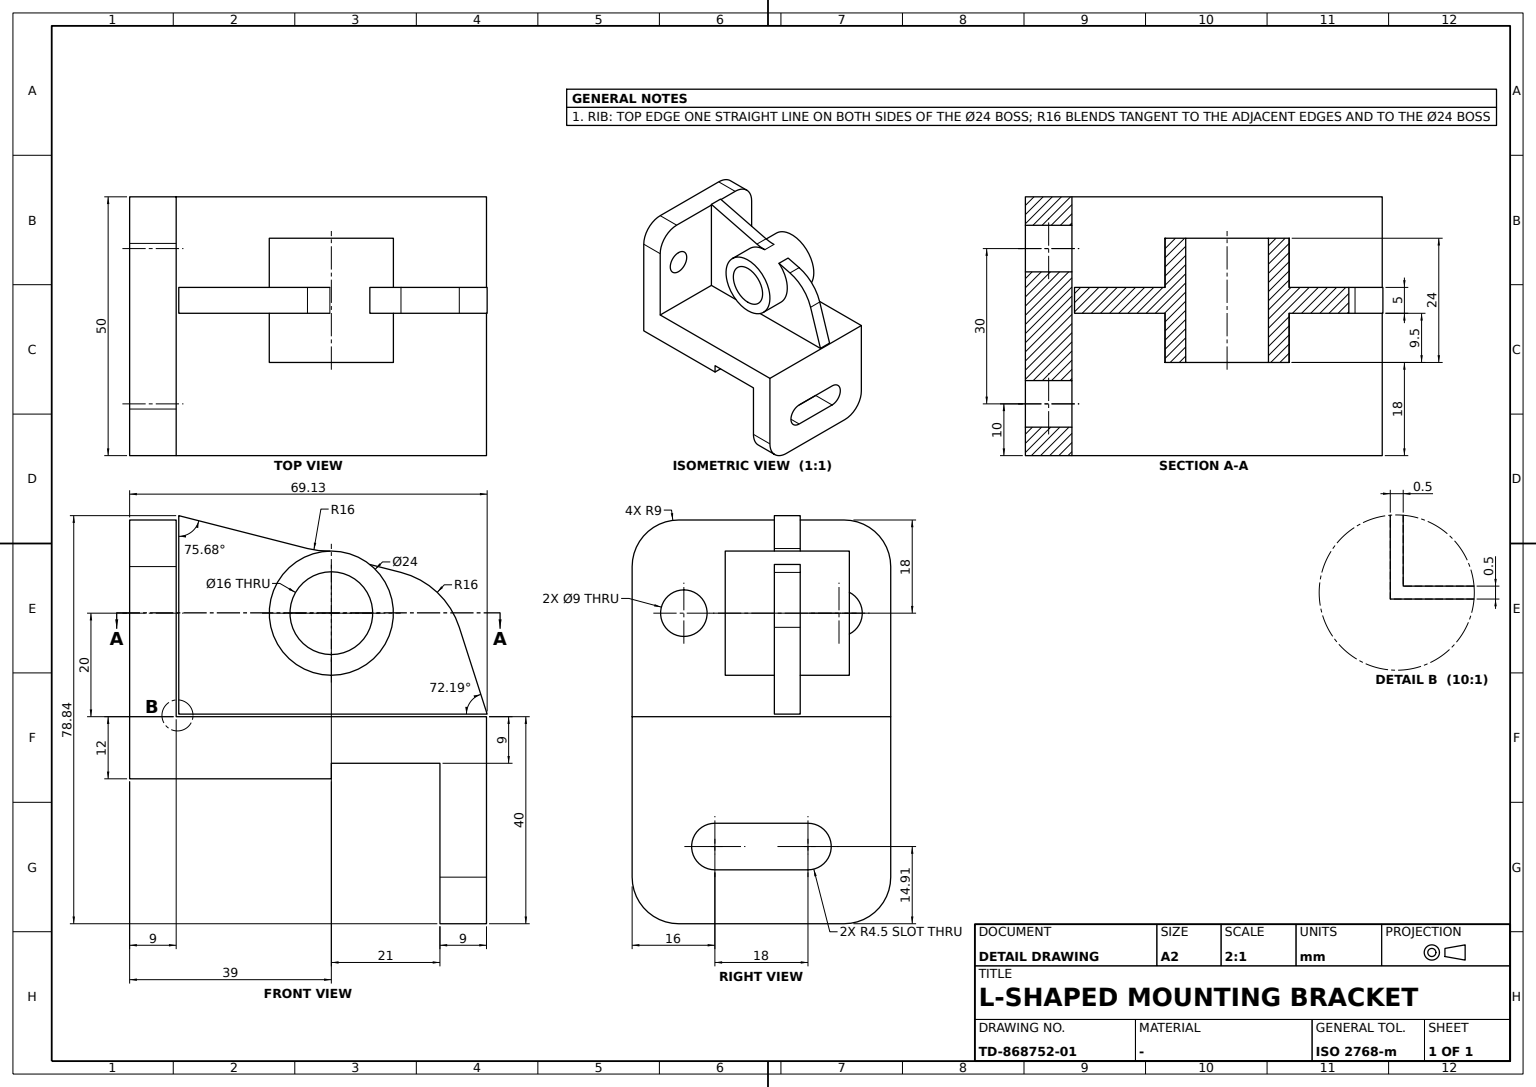
ISO-10303-21;
HEADER;
FILE_DESCRIPTION((''),'2;1');
FILE_NAME('','',(''),(''),'','','');
FILE_SCHEMA(('AUTOMOTIVE_DESIGN'));
ENDSEC;
DATA;
#1=APPLICATION_CONTEXT('');
#2=PRODUCT_CONTEXT('',#1,'mechanical');
#3=PRODUCT('','','',(#2));
#4=PRODUCT_DEFINITION_FORMATION('','',#3);
#5=PRODUCT_DEFINITION_CONTEXT('',#1,'design');
#6=PRODUCT_DEFINITION('','',#4,#5);
#7=PRODUCT_DEFINITION_SHAPE('','',#6);
#8=(LENGTH_UNIT()NAMED_UNIT(*)SI_UNIT(.MILLI.,.METRE.));
#9=(NAMED_UNIT(*)PLANE_ANGLE_UNIT()SI_UNIT($,.RADIAN.));
#10=(NAMED_UNIT(*)SI_UNIT($,.STERADIAN.)SOLID_ANGLE_UNIT());
#11=UNCERTAINTY_MEASURE_WITH_UNIT(LENGTH_MEASURE(0.005),#8,'distance_accuracy_value','');
#12=(GEOMETRIC_REPRESENTATION_CONTEXT(3)GLOBAL_UNCERTAINTY_ASSIGNED_CONTEXT((#11))GLOBAL_UNIT_ASSIGNED_CONTEXT((#8,#9,#10))REPRESENTATION_CONTEXT('',''));
#13=CARTESIAN_POINT('',(0.,-51.,12.));
#14=VERTEX_POINT('',#13);
#15=CARTESIAN_POINT('',(0.,-51.,41.));
#16=VERTEX_POINT('',#15);
#17=CARTESIAN_POINT('',(0.,-51.,0.));
#18=DIRECTION('',(0.,0.,1.));
#19=VECTOR('',#18,1000.);
#20=LINE('',#17,#19);
#21=EDGE_CURVE('',#14,#16,#20,.T.);
#22=ORIENTED_EDGE('',*,*,#21,.T.);
#23=CARTESIAN_POINT('',(9.,-51.,50.));
#24=VERTEX_POINT('',#23);
#25=CARTESIAN_POINT('',(9.,-51.,41.));
#26=DIRECTION('',(0.,1.,0.));
#27=AXIS2_PLACEMENT_3D('',#25,#26,#18);
#28=CIRCLE('',#27,9.);
#29=EDGE_CURVE('',#16,#24,#28,.T.);
#30=ORIENTED_EDGE('',*,*,#29,.T.);
#31=CARTESIAN_POINT('',(41.,-51.,50.));
#32=VERTEX_POINT('',#31);
#33=CARTESIAN_POINT('',(0.,-51.,50.));
#34=DIRECTION('',(1.,0.,0.));
#35=VECTOR('',#34,1000.);
#36=LINE('',#33,#35);
#37=EDGE_CURVE('',#24,#32,#36,.T.);
#38=ORIENTED_EDGE('',*,*,#37,.T.);
#39=CARTESIAN_POINT('',(50.,-51.,41.));
#40=VERTEX_POINT('',#39);
#41=CARTESIAN_POINT('',(41.,-51.,41.));
#42=AXIS2_PLACEMENT_3D('',#41,#26,#18);
#43=CIRCLE('',#42,9.);
#44=EDGE_CURVE('',#32,#40,#43,.T.);
#45=ORIENTED_EDGE('',*,*,#44,.T.);
#46=CARTESIAN_POINT('',(50.,-51.,12.));
#47=VERTEX_POINT('',#46);
#48=CARTESIAN_POINT('',(50.,-51.,0.));
#49=LINE('',#48,#19);
#50=EDGE_CURVE('',#47,#40,#49,.T.);
#51=ORIENTED_EDGE('',*,*,#50,.F.);
#52=LINE('',#13,#35);
#53=EDGE_CURVE('',#14,#47,#52,.T.);
#54=ORIENTED_EDGE('',*,*,#53,.F.);
#55=EDGE_LOOP('',(#22,#30,#38,#45,#51,#54));
#56=FACE_BOUND('',#55,.T.);
#57=CARTESIAN_POINT('',(10.,-51.,36.5));
#58=VERTEX_POINT('',#57);
#59=CARTESIAN_POINT('',(10.,-51.,32.));
#60=AXIS2_PLACEMENT_3D('',#59,#26,#18);
#61=CIRCLE('',#60,4.5);
#62=EDGE_CURVE('',#58,#58,#61,.T.);
#63=ORIENTED_EDGE('',*,*,#62,.F.);
#64=EDGE_LOOP('',(#63));
#65=FACE_BOUND('',#64,.T.);
#66=CARTESIAN_POINT('',(40.,-51.,36.5));
#67=VERTEX_POINT('',#66);
#68=CARTESIAN_POINT('',(40.,-51.,32.));
#69=AXIS2_PLACEMENT_3D('',#68,#26,#18);
#70=CIRCLE('',#69,4.5);
#71=EDGE_CURVE('',#67,#67,#70,.T.);
#72=ORIENTED_EDGE('',*,*,#71,.F.);
#73=EDGE_LOOP('',(#72));
#74=FACE_BOUND('',#73,.T.);
#75=AXIS2_PLACEMENT_3D('',#13,#26,#18);
#76=PLANE('',#75);
#77=ADVANCED_FACE('',(#56,#65,#74),#76,.T.);
#78=CARTESIAN_POINT('',(34.,9.,-8.585905426));
#79=VERTEX_POINT('',#78);
#80=CARTESIAN_POINT('',(34.,0.,-8.585905426));
#81=VERTEX_POINT('',#80);
#82=CARTESIAN_POINT('',(34.,-26.16,-8.585905426));
#83=VECTOR('',#26,1000.);
#84=LINE('',#82,#83);
#85=EDGE_CURVE('',#79,#81,#84,.F.);
#86=ORIENTED_EDGE('',*,*,#85,.F.);
#87=CARTESIAN_POINT('',(34.,9.,-17.585905426));
#88=VERTEX_POINT('',#87);
#89=CARTESIAN_POINT('',(34.,9.,-13.085905426));
#90=AXIS2_PLACEMENT_3D('',#89,#26,#18);
#91=CIRCLE('',#90,4.5);
#92=EDGE_CURVE('',#79,#88,#91,.T.);
#93=ORIENTED_EDGE('',*,*,#92,.T.);
#94=CARTESIAN_POINT('',(34.,0.,-17.585905426));
#95=VERTEX_POINT('',#94);
#96=CARTESIAN_POINT('',(34.,-26.16,-17.585905426));
#97=LINE('',#96,#83);
#98=EDGE_CURVE('',#88,#95,#97,.F.);
#99=ORIENTED_EDGE('',*,*,#98,.T.);
#100=CARTESIAN_POINT('',(34.,0.,-13.085905426));
#101=DIRECTION('',(0.,-1.,0.));
#102=DIRECTION('',(0.,0.,-1.));
#103=AXIS2_PLACEMENT_3D('',#100,#101,#102);
#104=CIRCLE('',#103,4.5);
#105=EDGE_CURVE('',#95,#81,#104,.T.);
#106=ORIENTED_EDGE('',*,*,#105,.T.);
#107=EDGE_LOOP('',(#86,#93,#99,#106));
#108=FACE_BOUND('',#107,.T.);
#109=CARTESIAN_POINT('',(34.,-26.16,-13.085905426));
#110=DIRECTION('',(-1.,0.,0.));
#111=AXIS2_PLACEMENT_3D('',#109,#26,#110);
#112=CYLINDRICAL_SURFACE('',#111,4.5);
#113=ADVANCED_FACE('',(#108),#112,.F.);
#114=ORIENTED_EDGE('',*,*,#62,.T.);
#115=EDGE_LOOP('',(#114));
#116=FACE_BOUND('',#115,.T.);
#117=CARTESIAN_POINT('',(10.,-60.,27.5));
#118=VERTEX_POINT('',#117);
#119=CARTESIAN_POINT('',(10.,-60.,32.));
#120=AXIS2_PLACEMENT_3D('',#119,#101,#102);
#121=CIRCLE('',#120,4.5);
#122=EDGE_CURVE('',#118,#118,#121,.T.);
#123=ORIENTED_EDGE('',*,*,#122,.T.);
#124=EDGE_LOOP('',(#123));
#125=FACE_BOUND('',#124,.T.);
#126=CARTESIAN_POINT('',(10.,-56.160000001,32.));
#127=AXIS2_PLACEMENT_3D('',#126,#26,#110);
#128=CYLINDRICAL_SURFACE('',#127,4.5);
#129=ADVANCED_FACE('',(#116,#125),#128,.F.);
#130=CARTESIAN_POINT('',(0.,-21.,3.));
#131=VERTEX_POINT('',#130);
#132=CARTESIAN_POINT('',(0.,0.,3.));
#133=VERTEX_POINT('',#132);
#134=LINE('',#132,#83);
#135=EDGE_CURVE('',#131,#133,#134,.T.);
#136=ORIENTED_EDGE('',*,*,#135,.T.);
#137=CARTESIAN_POINT('',(50.,0.,3.));
#138=VERTEX_POINT('',#137);
#139=LINE('',#132,#35);
#140=EDGE_CURVE('',#133,#138,#139,.T.);
#141=ORIENTED_EDGE('',*,*,#140,.T.);
#142=CARTESIAN_POINT('',(50.,-21.,3.));
#143=VERTEX_POINT('',#142);
#144=LINE('',#137,#83);
#145=EDGE_CURVE('',#143,#138,#144,.T.);
#146=ORIENTED_EDGE('',*,*,#145,.F.);
#147=LINE('',#130,#35);
#148=EDGE_CURVE('',#131,#143,#147,.T.);
#149=ORIENTED_EDGE('',*,*,#148,.F.);
#150=EDGE_LOOP('',(#136,#141,#146,#149));
#151=FACE_BOUND('',#150,.T.);
#152=AXIS2_PLACEMENT_3D('',#130,#102,#26);
#153=PLANE('',#152);
#154=ADVANCED_FACE('',(#151),#153,.T.);
#155=ORIENTED_EDGE('',*,*,#92,.F.);
#156=CARTESIAN_POINT('',(16.,9.,-8.585905426));
#157=VERTEX_POINT('',#156);
#158=VECTOR('',#110,1000.);
#159=LINE('',#78,#158);
#160=EDGE_CURVE('',#79,#157,#159,.T.);
#161=ORIENTED_EDGE('',*,*,#160,.T.);
#162=CARTESIAN_POINT('',(16.,9.,-17.585905426));
#163=VERTEX_POINT('',#162);
#164=CARTESIAN_POINT('',(16.,9.,-13.085905426));
#165=AXIS2_PLACEMENT_3D('',#164,#26,#18);
#166=CIRCLE('',#165,4.5);
#167=EDGE_CURVE('',#163,#157,#166,.T.);
#168=ORIENTED_EDGE('',*,*,#167,.F.);
#169=LINE('',#87,#158);
#170=EDGE_CURVE('',#88,#163,#169,.T.);
#171=ORIENTED_EDGE('',*,*,#170,.F.);
#172=EDGE_LOOP('',(#155,#161,#168,#171));
#173=FACE_BOUND('',#172,.T.);
#174=CARTESIAN_POINT('',(9.,9.,-28.));
#175=VERTEX_POINT('',#174);
#176=CARTESIAN_POINT('',(0.,9.,-19.));
#177=VERTEX_POINT('',#176);
#178=CARTESIAN_POINT('',(9.,9.,-19.));
#179=AXIS2_PLACEMENT_3D('',#178,#26,#18);
#180=CIRCLE('',#179,9.);
#181=EDGE_CURVE('',#175,#177,#180,.T.);
#182=ORIENTED_EDGE('',*,*,#181,.T.);
#183=CARTESIAN_POINT('',(0.,9.,12.));
#184=VERTEX_POINT('',#183);
#185=CARTESIAN_POINT('',(0.,9.,0.));
#186=LINE('',#185,#19);
#187=EDGE_CURVE('',#177,#184,#186,.T.);
#188=ORIENTED_EDGE('',*,*,#187,.T.);
#189=CARTESIAN_POINT('',(50.,9.,12.));
#190=VERTEX_POINT('',#189);
#191=LINE('',#183,#35);
#192=EDGE_CURVE('',#184,#190,#191,.T.);
#193=ORIENTED_EDGE('',*,*,#192,.T.);
#194=CARTESIAN_POINT('',(50.,9.,-19.));
#195=VERTEX_POINT('',#194);
#196=CARTESIAN_POINT('',(50.,9.,0.));
#197=LINE('',#196,#19);
#198=EDGE_CURVE('',#195,#190,#197,.T.);
#199=ORIENTED_EDGE('',*,*,#198,.F.);
#200=CARTESIAN_POINT('',(41.,9.,-28.));
#201=VERTEX_POINT('',#200);
#202=CARTESIAN_POINT('',(41.,9.,-19.));
#203=AXIS2_PLACEMENT_3D('',#202,#26,#18);
#204=CIRCLE('',#203,9.);
#205=EDGE_CURVE('',#195,#201,#204,.T.);
#206=ORIENTED_EDGE('',*,*,#205,.T.);
#207=CARTESIAN_POINT('',(0.,9.,-28.));
#208=LINE('',#207,#35);
#209=EDGE_CURVE('',#175,#201,#208,.T.);
#210=ORIENTED_EDGE('',*,*,#209,.F.);
#211=EDGE_LOOP('',(#182,#188,#193,#199,#206,#210));
#212=FACE_BOUND('',#211,.T.);
#213=AXIS2_PLACEMENT_3D('',#207,#26,#18);
#214=PLANE('',#213);
#215=ADVANCED_FACE('',(#173,#212),#214,.T.);
#216=CARTESIAN_POINT('',(0.,0.,12.));
#217=VECTOR('',#101,1000.);
#218=LINE('',#216,#217);
#219=EDGE_CURVE('',#184,#14,#218,.T.);
#220=ORIENTED_EDGE('',*,*,#219,.F.);
#221=ORIENTED_EDGE('',*,*,#187,.F.);
#222=CARTESIAN_POINT('',(0.,0.,-19.));
#223=VERTEX_POINT('',#222);
#224=CARTESIAN_POINT('',(0.,-25.5,-19.));
#225=LINE('',#224,#83);
#226=EDGE_CURVE('',#223,#177,#225,.T.);
#227=ORIENTED_EDGE('',*,*,#226,.F.);
#228=CARTESIAN_POINT('',(0.,0.,0.));
#229=VECTOR('',#102,1000.);
#230=LINE('',#228,#229);
#231=EDGE_CURVE('',#133,#223,#230,.T.);
#232=ORIENTED_EDGE('',*,*,#231,.F.);
#233=ORIENTED_EDGE('',*,*,#135,.F.);
#234=CARTESIAN_POINT('',(0.,-21.,0.));
#235=VERTEX_POINT('',#234);
#236=LINE('',#234,#19);
#237=EDGE_CURVE('',#235,#131,#236,.T.);
#238=ORIENTED_EDGE('',*,*,#237,.F.);
#239=CARTESIAN_POINT('',(0.,-60.,0.));
#240=VERTEX_POINT('',#239);
#241=LINE('',#228,#83);
#242=EDGE_CURVE('',#240,#235,#241,.T.);
#243=ORIENTED_EDGE('',*,*,#242,.F.);
#244=CARTESIAN_POINT('',(0.,-60.,41.));
#245=VERTEX_POINT('',#244);
#246=LINE('',#239,#229);
#247=EDGE_CURVE('',#245,#240,#246,.T.);
#248=ORIENTED_EDGE('',*,*,#247,.F.);
#249=CARTESIAN_POINT('',(0.,-25.5,41.));
#250=LINE('',#249,#217);
#251=EDGE_CURVE('',#16,#245,#250,.T.);
#252=ORIENTED_EDGE('',*,*,#251,.F.);
#253=ORIENTED_EDGE('',*,*,#21,.F.);
#254=EDGE_LOOP('',(#220,#221,#227,#232,#233,#238,#243,#248,#252,#253));
#255=FACE_BOUND('',#254,.T.);
#256=AXIS2_PLACEMENT_3D('',#228,#34,#26);
#257=PLANE('',#256);
#258=ADVANCED_FACE('',(#255),#257,.F.);
#259=CARTESIAN_POINT('',(16.,0.,-17.585905426));
#260=VERTEX_POINT('',#259);
#261=CARTESIAN_POINT('',(0.,0.,-17.585905426));
#262=LINE('',#261,#158);
#263=EDGE_CURVE('',#95,#260,#262,.T.);
#264=ORIENTED_EDGE('',*,*,#263,.T.);
#265=CARTESIAN_POINT('',(16.,0.,-8.585905426));
#266=VERTEX_POINT('',#265);
#267=CARTESIAN_POINT('',(16.,0.,-13.085905426));
#268=AXIS2_PLACEMENT_3D('',#267,#101,#102);
#269=CIRCLE('',#268,4.5);
#270=EDGE_CURVE('',#266,#260,#269,.T.);
#271=ORIENTED_EDGE('',*,*,#270,.F.);
#272=CARTESIAN_POINT('',(0.,0.,-8.585905426));
#273=LINE('',#272,#158);
#274=EDGE_CURVE('',#81,#266,#273,.T.);
#275=ORIENTED_EDGE('',*,*,#274,.F.);
#276=ORIENTED_EDGE('',*,*,#105,.F.);
#277=EDGE_LOOP('',(#264,#271,#275,#276));
#278=FACE_BOUND('',#277,.T.);
#279=ORIENTED_EDGE('',*,*,#231,.T.);
#280=CARTESIAN_POINT('',(9.,0.,-28.));
#281=VERTEX_POINT('',#280);
#282=CARTESIAN_POINT('',(9.,0.,-19.));
#283=AXIS2_PLACEMENT_3D('',#282,#101,#102);
#284=CIRCLE('',#283,9.);
#285=EDGE_CURVE('',#223,#281,#284,.T.);
#286=ORIENTED_EDGE('',*,*,#285,.T.);
#287=CARTESIAN_POINT('',(41.,0.,-28.));
#288=VERTEX_POINT('',#287);
#289=CARTESIAN_POINT('',(0.,0.,-28.));
#290=LINE('',#289,#35);
#291=EDGE_CURVE('',#281,#288,#290,.T.);
#292=ORIENTED_EDGE('',*,*,#291,.T.);
#293=CARTESIAN_POINT('',(50.,0.,-19.));
#294=VERTEX_POINT('',#293);
#295=CARTESIAN_POINT('',(41.,0.,-19.));
#296=AXIS2_PLACEMENT_3D('',#295,#101,#102);
#297=CIRCLE('',#296,9.);
#298=EDGE_CURVE('',#288,#294,#297,.T.);
#299=ORIENTED_EDGE('',*,*,#298,.T.);
#300=CARTESIAN_POINT('',(50.,0.,0.));
#301=LINE('',#300,#229);
#302=EDGE_CURVE('',#138,#294,#301,.T.);
#303=ORIENTED_EDGE('',*,*,#302,.F.);
#304=ORIENTED_EDGE('',*,*,#140,.F.);
#305=EDGE_LOOP('',(#279,#286,#292,#299,#303,#304));
#306=FACE_BOUND('',#305,.T.);
#307=AXIS2_PLACEMENT_3D('',#132,#101,#102);
#308=PLANE('',#307);
#309=ADVANCED_FACE('',(#278,#306),#308,.T.);
#310=ORIENTED_EDGE('',*,*,#237,.T.);
#311=ORIENTED_EDGE('',*,*,#148,.T.);
#312=CARTESIAN_POINT('',(50.,-21.,0.));
#313=VERTEX_POINT('',#312);
#314=LINE('',#312,#19);
#315=EDGE_CURVE('',#313,#143,#314,.T.);
#316=ORIENTED_EDGE('',*,*,#315,.F.);
#317=LINE('',#234,#35);
#318=EDGE_CURVE('',#235,#313,#317,.T.);
#319=ORIENTED_EDGE('',*,*,#318,.F.);
#320=EDGE_LOOP('',(#310,#311,#316,#319));
#321=FACE_BOUND('',#320,.T.);
#322=AXIS2_PLACEMENT_3D('',#234,#26,#18);
#323=PLANE('',#322);
#324=ADVANCED_FACE('',(#321),#323,.T.);
#325=CARTESIAN_POINT('',(9.,-60.,50.));
#326=VERTEX_POINT('',#325);
#327=CARTESIAN_POINT('',(9.,-25.5,50.));
#328=LINE('',#327,#217);
#329=EDGE_CURVE('',#24,#326,#328,.T.);
#330=ORIENTED_EDGE('',*,*,#329,.T.);
#331=CARTESIAN_POINT('',(41.,-60.,50.));
#332=VERTEX_POINT('',#331);
#333=CARTESIAN_POINT('',(0.,-60.,50.));
#334=LINE('',#333,#35);
#335=EDGE_CURVE('',#326,#332,#334,.T.);
#336=ORIENTED_EDGE('',*,*,#335,.T.);
#337=CARTESIAN_POINT('',(41.,-25.5,50.));
#338=LINE('',#337,#217);
#339=EDGE_CURVE('',#32,#332,#338,.T.);
#340=ORIENTED_EDGE('',*,*,#339,.F.);
#341=ORIENTED_EDGE('',*,*,#37,.F.);
#342=EDGE_LOOP('',(#330,#336,#340,#341));
#343=FACE_BOUND('',#342,.T.);
#344=AXIS2_PLACEMENT_3D('',#33,#18,#101);
#345=PLANE('',#344);
#346=ADVANCED_FACE('',(#343),#345,.T.);
#347=CARTESIAN_POINT('',(41.,-25.5,-28.));
#348=LINE('',#347,#83);
#349=EDGE_CURVE('',#288,#201,#348,.T.);
#350=ORIENTED_EDGE('',*,*,#349,.T.);
#351=ORIENTED_EDGE('',*,*,#205,.F.);
#352=CARTESIAN_POINT('',(50.,-25.5,-19.));
#353=LINE('',#352,#83);
#354=EDGE_CURVE('',#294,#195,#353,.T.);
#355=ORIENTED_EDGE('',*,*,#354,.F.);
#356=ORIENTED_EDGE('',*,*,#298,.F.);
#357=EDGE_LOOP('',(#350,#351,#355,#356));
#358=FACE_BOUND('',#357,.T.);
#359=CARTESIAN_POINT('',(41.,-25.5,-19.));
#360=AXIS2_PLACEMENT_3D('',#359,#26,#102);
#361=CYLINDRICAL_SURFACE('',#360,9.);
#362=ADVANCED_FACE('',(#358),#361,.T.);
#363=ORIENTED_EDGE('',*,*,#209,.T.);
#364=ORIENTED_EDGE('',*,*,#349,.F.);
#365=ORIENTED_EDGE('',*,*,#291,.F.);
#366=CARTESIAN_POINT('',(9.,-25.5,-28.));
#367=LINE('',#366,#83);
#368=EDGE_CURVE('',#281,#175,#367,.T.);
#369=ORIENTED_EDGE('',*,*,#368,.T.);
#370=EDGE_LOOP('',(#363,#364,#365,#369));
#371=FACE_BOUND('',#370,.T.);
#372=AXIS2_PLACEMENT_3D('',#289,#102,#26);
#373=PLANE('',#372);
#374=ADVANCED_FACE('',(#371),#373,.T.);
#375=CARTESIAN_POINT('',(50.,-60.,41.));
#376=VERTEX_POINT('',#375);
#377=CARTESIAN_POINT('',(41.,-60.,41.));
#378=AXIS2_PLACEMENT_3D('',#377,#101,#102);
#379=CIRCLE('',#378,9.);
#380=EDGE_CURVE('',#376,#332,#379,.T.);
#381=ORIENTED_EDGE('',*,*,#380,.F.);
#382=CARTESIAN_POINT('',(50.,-25.5,41.));
#383=LINE('',#382,#217);
#384=EDGE_CURVE('',#40,#376,#383,.T.);
#385=ORIENTED_EDGE('',*,*,#384,.F.);
#386=ORIENTED_EDGE('',*,*,#44,.F.);
#387=ORIENTED_EDGE('',*,*,#339,.T.);
#388=EDGE_LOOP('',(#381,#385,#386,#387));
#389=FACE_BOUND('',#388,.T.);
#390=CARTESIAN_POINT('',(41.,-25.5,41.));
#391=AXIS2_PLACEMENT_3D('',#390,#101,#18);
#392=CYLINDRICAL_SURFACE('',#391,9.);
#393=ADVANCED_FACE('',(#389),#392,.T.);
#394=CARTESIAN_POINT('',(40.,-60.,27.5));
#395=VERTEX_POINT('',#394);
#396=CARTESIAN_POINT('',(40.,-60.,32.));
#397=AXIS2_PLACEMENT_3D('',#396,#101,#102);
#398=CIRCLE('',#397,4.5);
#399=EDGE_CURVE('',#395,#395,#398,.T.);
#400=ORIENTED_EDGE('',*,*,#399,.T.);
#401=EDGE_LOOP('',(#400));
#402=FACE_BOUND('',#401,.T.);
#403=ORIENTED_EDGE('',*,*,#71,.T.);
#404=EDGE_LOOP('',(#403));
#405=FACE_BOUND('',#404,.T.);
#406=CARTESIAN_POINT('',(40.,-56.160000001,32.));
#407=AXIS2_PLACEMENT_3D('',#406,#26,#110);
#408=CYLINDRICAL_SURFACE('',#407,4.5);
#409=ADVANCED_FACE('',(#402,#405),#408,.F.);
#410=ORIENTED_EDGE('',*,*,#368,.F.);
#411=ORIENTED_EDGE('',*,*,#285,.F.);
#412=ORIENTED_EDGE('',*,*,#226,.T.);
#413=ORIENTED_EDGE('',*,*,#181,.F.);
#414=EDGE_LOOP('',(#410,#411,#412,#413));
#415=FACE_BOUND('',#414,.T.);
#416=CARTESIAN_POINT('',(9.,-25.5,-19.));
#417=AXIS2_PLACEMENT_3D('',#416,#26,#110);
#418=CYLINDRICAL_SURFACE('',#417,9.);
#419=ADVANCED_FACE('',(#415),#418,.T.);
#420=CARTESIAN_POINT('',(50.,-60.,0.));
#421=VERTEX_POINT('',#420);
#422=LINE('',#300,#83);
#423=EDGE_CURVE('',#421,#313,#422,.T.);
#424=ORIENTED_EDGE('',*,*,#423,.F.);
#425=LINE('',#239,#35);
#426=EDGE_CURVE('',#240,#421,#425,.T.);
#427=ORIENTED_EDGE('',*,*,#426,.F.);
#428=ORIENTED_EDGE('',*,*,#242,.T.);
#429=ORIENTED_EDGE('',*,*,#318,.T.);
#430=EDGE_LOOP('',(#424,#427,#428,#429));
#431=FACE_BOUND('',#430,.T.);
#432=AXIS2_PLACEMENT_3D('',#239,#102,#26);
#433=PLANE('',#432);
#434=ADVANCED_FACE('',(#431),#433,.T.);
#435=ORIENTED_EDGE('',*,*,#274,.T.);
#436=CARTESIAN_POINT('',(16.,-26.16,-8.585905426));
#437=LINE('',#436,#83);
#438=EDGE_CURVE('',#157,#266,#437,.F.);
#439=ORIENTED_EDGE('',*,*,#438,.F.);
#440=ORIENTED_EDGE('',*,*,#160,.F.);
#441=ORIENTED_EDGE('',*,*,#85,.T.);
#442=EDGE_LOOP('',(#435,#439,#440,#441));
#443=FACE_BOUND('',#442,.T.);
#444=AXIS2_PLACEMENT_3D('',#78,#18,#110);
#445=PLANE('',#444);
#446=ADVANCED_FACE('',(#443),#445,.F.);
#447=ORIENTED_EDGE('',*,*,#29,.F.);
#448=ORIENTED_EDGE('',*,*,#251,.T.);
#449=CARTESIAN_POINT('',(9.,-60.,41.));
#450=AXIS2_PLACEMENT_3D('',#449,#101,#102);
#451=CIRCLE('',#450,9.);
#452=EDGE_CURVE('',#326,#245,#451,.T.);
#453=ORIENTED_EDGE('',*,*,#452,.F.);
#454=ORIENTED_EDGE('',*,*,#329,.F.);
#455=EDGE_LOOP('',(#447,#448,#453,#454));
#456=FACE_BOUND('',#455,.T.);
#457=CARTESIAN_POINT('',(9.,-25.5,41.));
#458=AXIS2_PLACEMENT_3D('',#457,#101,#110);
#459=CYLINDRICAL_SURFACE('',#458,9.);
#460=ADVANCED_FACE('',(#456),#459,.T.);
#461=ORIENTED_EDGE('',*,*,#399,.F.);
#462=EDGE_LOOP('',(#461));
#463=FACE_BOUND('',#462,.T.);
#464=ORIENTED_EDGE('',*,*,#335,.F.);
#465=ORIENTED_EDGE('',*,*,#452,.T.);
#466=ORIENTED_EDGE('',*,*,#247,.T.);
#467=ORIENTED_EDGE('',*,*,#426,.T.);
#468=LINE('',#420,#229);
#469=EDGE_CURVE('',#376,#421,#468,.T.);
#470=ORIENTED_EDGE('',*,*,#469,.F.);
#471=ORIENTED_EDGE('',*,*,#380,.T.);
#472=EDGE_LOOP('',(#464,#465,#466,#467,#470,#471));
#473=FACE_BOUND('',#472,.T.);
#474=ORIENTED_EDGE('',*,*,#122,.F.);
#475=EDGE_LOOP('',(#474));
#476=FACE_BOUND('',#475,.T.);
#477=AXIS2_PLACEMENT_3D('',#333,#101,#102);
#478=PLANE('',#477);
#479=ADVANCED_FACE('',(#463,#473,#476),#478,.T.);
#480=ORIENTED_EDGE('',*,*,#438,.T.);
#481=ORIENTED_EDGE('',*,*,#270,.T.);
#482=CARTESIAN_POINT('',(16.,-26.16,-17.585905426));
#483=LINE('',#482,#83);
#484=EDGE_CURVE('',#163,#260,#483,.F.);
#485=ORIENTED_EDGE('',*,*,#484,.F.);
#486=ORIENTED_EDGE('',*,*,#167,.T.);
#487=EDGE_LOOP('',(#480,#481,#485,#486));
#488=FACE_BOUND('',#487,.T.);
#489=CARTESIAN_POINT('',(16.,-26.16,-13.085905426));
#490=AXIS2_PLACEMENT_3D('',#489,#26,#110);
#491=CYLINDRICAL_SURFACE('',#490,4.5);
#492=ADVANCED_FACE('',(#488),#491,.F.);
#493=CARTESIAN_POINT('',(50.,0.,12.));
#494=LINE('',#493,#217);
#495=EDGE_CURVE('',#190,#47,#494,.T.);
#496=ORIENTED_EDGE('',*,*,#495,.F.);
#497=ORIENTED_EDGE('',*,*,#192,.F.);
#498=ORIENTED_EDGE('',*,*,#219,.T.);
#499=ORIENTED_EDGE('',*,*,#53,.T.);
#500=EDGE_LOOP('',(#496,#497,#498,#499));
#501=FACE_BOUND('',#500,.T.);
#502=AXIS2_PLACEMENT_3D('',#183,#18,#101);
#503=PLANE('',#502);
#504=ADVANCED_FACE('',(#501),#503,.T.);
#505=ORIENTED_EDGE('',*,*,#263,.F.);
#506=ORIENTED_EDGE('',*,*,#98,.F.);
#507=ORIENTED_EDGE('',*,*,#170,.T.);
#508=ORIENTED_EDGE('',*,*,#484,.T.);
#509=EDGE_LOOP('',(#505,#506,#507,#508));
#510=FACE_BOUND('',#509,.T.);
#511=AXIS2_PLACEMENT_3D('',#87,#18,#110);
#512=PLANE('',#511);
#513=ADVANCED_FACE('',(#510),#512,.T.);
#514=ORIENTED_EDGE('',*,*,#423,.T.);
#515=ORIENTED_EDGE('',*,*,#315,.T.);
#516=ORIENTED_EDGE('',*,*,#145,.T.);
#517=ORIENTED_EDGE('',*,*,#302,.T.);
#518=ORIENTED_EDGE('',*,*,#354,.T.);
#519=ORIENTED_EDGE('',*,*,#198,.T.);
#520=ORIENTED_EDGE('',*,*,#495,.T.);
#521=ORIENTED_EDGE('',*,*,#50,.T.);
#522=ORIENTED_EDGE('',*,*,#384,.T.);
#523=ORIENTED_EDGE('',*,*,#469,.T.);
#524=EDGE_LOOP('',(#514,#515,#516,#517,#518,#519,#520,#521,#522,#523));
#525=FACE_BOUND('',#524,.T.);
#526=AXIS2_PLACEMENT_3D('',#300,#34,#26);
#527=PLANE('',#526);
#528=ADVANCED_FACE('',(#525),#527,.T.);
#529=CLOSED_SHELL('',(#77,#113,#129,#154,#215,#258,#309,#324,#346,#362,#374,#393,#409,#419,#434,#446,#460,#479,#492,#504,#513,#528));
#530=MANIFOLD_SOLID_BREP('',#529);
#531=CARTESIAN_POINT('',(22.5,-21.28181978,43.996690277));
#532=VERTEX_POINT('',#531);
#533=CARTESIAN_POINT('',(22.5,-13.554664906,41.411003418));
#534=VERTEX_POINT('',#533);
#535=CARTESIAN_POINT('',(22.5,-21.,32.));
#536=AXIS2_PLACEMENT_3D('',#535,#34,#102);
#537=CIRCLE('',#536,12.);
#538=EDGE_CURVE('',#532,#534,#537,.T.);
#539=ORIENTED_EDGE('',*,*,#538,.F.);
#540=CARTESIAN_POINT('',(22.5,-25.614715099,44.4893396));
#541=VERTEX_POINT('',#540);
#542=CARTESIAN_POINT('',(22.5,-21.657579487,59.992277314));
#543=AXIS2_PLACEMENT_3D('',#542,#34,#102);
#544=CIRCLE('',#543,16.);
#545=EDGE_CURVE('',#541,#532,#544,.T.);
#546=ORIENTED_EDGE('',*,*,#545,.F.);
#547=CARTESIAN_POINT('',(22.5,-50.5,50.841325844));
#548=VERTEX_POINT('',#547);
#549=CARTESIAN_POINT('',(22.5,1.036463778,37.686607694));
#550=DIRECTION('',(0.,-0.968933607,0.247320976));
#551=VECTOR('',#550,1000.);
#552=LINE('',#549,#551);
#553=EDGE_CURVE('',#541,#548,#552,.T.);
#554=ORIENTED_EDGE('',*,*,#553,.T.);
#555=CARTESIAN_POINT('',(22.5,-50.5,12.5));
#556=VERTEX_POINT('',#555);
#557=LINE('',#547,#229);
#558=EDGE_CURVE('',#548,#556,#557,.T.);
#559=ORIENTED_EDGE('',*,*,#558,.T.);
#560=CARTESIAN_POINT('',(22.5,9.128271653,12.5));
#561=VERTEX_POINT('',#560);
#562=LINE('',#555,#83);
#563=EDGE_CURVE('',#556,#561,#562,.T.);
#564=ORIENTED_EDGE('',*,*,#563,.T.);
#565=CARTESIAN_POINT('',(22.5,3.742012558,29.265301013));
#566=VERTEX_POINT('',#565);
#567=DIRECTION('',(0.,-0.305875989,0.952071362));
#568=VECTOR('',#567,1000.);
#569=LINE('',#560,#568);
#570=EDGE_CURVE('',#561,#566,#569,.T.);
#571=ORIENTED_EDGE('',*,*,#570,.T.);
#572=CARTESIAN_POINT('',(22.5,-7.533993629,39.874222896));
#573=VERTEX_POINT('',#572);
#574=CARTESIAN_POINT('',(22.5,-11.49112924,24.371285182));
#575=AXIS2_PLACEMENT_3D('',#574,#34,#102);
#576=CIRCLE('',#575,16.);
#577=EDGE_CURVE('',#566,#573,#576,.T.);
#578=ORIENTED_EDGE('',*,*,#577,.T.);
#579=EDGE_CURVE('',#573,#534,#552,.T.);
#580=ORIENTED_EDGE('',*,*,#579,.T.);
#581=EDGE_LOOP('',(#539,#546,#554,#559,#564,#571,#578,#580));
#582=FACE_BOUND('',#581,.T.);
#583=CARTESIAN_POINT('',(22.5,0.,0.));
#584=AXIS2_PLACEMENT_3D('',#583,#34,#26);
#585=PLANE('',#584);
#586=ADVANCED_FACE('',(#582),#585,.T.);
#587=ORIENTED_EDGE('',*,*,#545,.T.);
#588=CARTESIAN_POINT('',(17.5,-21.28181978,43.996690277));
#589=VERTEX_POINT('',#588);
#590=CARTESIAN_POINT('',(20.,-21.28181978,43.996690277));
#591=LINE('',#590,#35);
#592=EDGE_CURVE('',#589,#532,#591,.T.);
#593=ORIENTED_EDGE('',*,*,#592,.F.);
#594=CARTESIAN_POINT('',(17.5,-25.614715099,44.4893396));
#595=VERTEX_POINT('',#594);
#596=CARTESIAN_POINT('',(17.5,-21.657579487,59.992277314));
#597=AXIS2_PLACEMENT_3D('',#596,#34,#102);
#598=CIRCLE('',#597,16.);
#599=EDGE_CURVE('',#595,#589,#598,.T.);
#600=ORIENTED_EDGE('',*,*,#599,.F.);
#601=CARTESIAN_POINT('',(20.,-25.614715099,44.4893396));
#602=LINE('',#601,#35);
#603=EDGE_CURVE('',#595,#541,#602,.T.);
#604=ORIENTED_EDGE('',*,*,#603,.T.);
#605=EDGE_LOOP('',(#587,#593,#600,#604));
#606=FACE_BOUND('',#605,.T.);
#607=CARTESIAN_POINT('',(20.,-21.657579487,59.992277314));
#608=DIRECTION('',(0.,0.023484982,-0.99972419));
#609=AXIS2_PLACEMENT_3D('',#607,#34,#608);
#610=CYLINDRICAL_SURFACE('',#609,16.);
#611=ADVANCED_FACE('',(#606),#610,.F.);
#612=CARTESIAN_POINT('',(32.,-21.,24.));
#613=VERTEX_POINT('',#612);
#614=CARTESIAN_POINT('',(32.,-21.,32.));
#615=AXIS2_PLACEMENT_3D('',#614,#34,#102);
#616=CIRCLE('',#615,8.);
#617=EDGE_CURVE('',#613,#613,#616,.T.);
#618=ORIENTED_EDGE('',*,*,#617,.T.);
#619=EDGE_LOOP('',(#618));
#620=FACE_BOUND('',#619,.T.);
#621=CARTESIAN_POINT('',(8.,-21.,24.));
#622=VERTEX_POINT('',#621);
#623=CARTESIAN_POINT('',(8.,-21.,32.));
#624=AXIS2_PLACEMENT_3D('',#623,#34,#102);
#625=CIRCLE('',#624,8.);
#626=EDGE_CURVE('',#622,#622,#625,.T.);
#627=ORIENTED_EDGE('',*,*,#626,.F.);
#628=EDGE_LOOP('',(#627));
#629=FACE_BOUND('',#628,.T.);
#630=CARTESIAN_POINT('',(20.,-21.,32.));
#631=AXIS2_PLACEMENT_3D('',#630,#34,#26);
#632=CYLINDRICAL_SURFACE('',#631,8.);
#633=ADVANCED_FACE('',(#620,#629),#632,.F.);
#634=CARTESIAN_POINT('',(17.5,3.742012558,29.265301013));
#635=VERTEX_POINT('',#634);
#636=CARTESIAN_POINT('',(17.5,-7.533993629,39.874222896));
#637=VERTEX_POINT('',#636);
#638=CARTESIAN_POINT('',(17.5,-11.49112924,24.371285182));
#639=AXIS2_PLACEMENT_3D('',#638,#34,#102);
#640=CIRCLE('',#639,16.);
#641=EDGE_CURVE('',#635,#637,#640,.T.);
#642=ORIENTED_EDGE('',*,*,#641,.T.);
#643=CARTESIAN_POINT('',(20.,-7.533993629,39.874222896));
#644=LINE('',#643,#158);
#645=EDGE_CURVE('',#573,#637,#644,.T.);
#646=ORIENTED_EDGE('',*,*,#645,.F.);
#647=ORIENTED_EDGE('',*,*,#577,.F.);
#648=CARTESIAN_POINT('',(20.,3.742012558,29.265301013));
#649=LINE('',#648,#158);
#650=EDGE_CURVE('',#566,#635,#649,.T.);
#651=ORIENTED_EDGE('',*,*,#650,.T.);
#652=EDGE_LOOP('',(#642,#646,#647,#651));
#653=FACE_BOUND('',#652,.T.);
#654=CARTESIAN_POINT('',(20.,-11.49112924,24.371285182));
#655=DIRECTION('',(0.,0.952071362,0.305875989));
#656=AXIS2_PLACEMENT_3D('',#654,#110,#655);
#657=CYLINDRICAL_SURFACE('',#656,16.);
#658=ADVANCED_FACE('',(#653),#657,.T.);
#659=ORIENTED_EDGE('',*,*,#579,.F.);
#660=ORIENTED_EDGE('',*,*,#645,.T.);
#661=CARTESIAN_POINT('',(17.5,-13.554664906,41.411003418));
#662=VERTEX_POINT('',#661);
#663=CARTESIAN_POINT('',(17.5,1.036463778,37.686607694));
#664=LINE('',#663,#551);
#665=EDGE_CURVE('',#637,#662,#664,.T.);
#666=ORIENTED_EDGE('',*,*,#665,.T.);
#667=LINE('',#533,#35);
#668=EDGE_CURVE('',#534,#662,#667,.F.);
#669=ORIENTED_EDGE('',*,*,#668,.F.);
#670=EDGE_LOOP('',(#659,#660,#666,#669));
#671=FACE_BOUND('',#670,.T.);
#672=CARTESIAN_POINT('',(20.,1.036463778,37.686607694));
#673=DIRECTION('',(0.,-0.247320976,-0.968933607));
#674=AXIS2_PLACEMENT_3D('',#672,#673,#550);
#675=PLANE('',#674);
#676=ADVANCED_FACE('',(#671),#675,.F.);
#677=CARTESIAN_POINT('',(8.,-21.,20.));
#678=VERTEX_POINT('',#677);
#679=CIRCLE('',#624,12.);
#680=EDGE_CURVE('',#678,#678,#679,.T.);
#681=ORIENTED_EDGE('',*,*,#680,.T.);
#682=EDGE_LOOP('',(#681));
#683=FACE_BOUND('',#682,.T.);
#684=CARTESIAN_POINT('',(32.,-21.,20.));
#685=VERTEX_POINT('',#684);
#686=CIRCLE('',#615,12.);
#687=EDGE_CURVE('',#685,#685,#686,.T.);
#688=ORIENTED_EDGE('',*,*,#687,.F.);
#689=EDGE_LOOP('',(#688));
#690=FACE_BOUND('',#689,.T.);
#691=ORIENTED_EDGE('',*,*,#668,.T.);
#692=CARTESIAN_POINT('',(17.5,-21.,32.));
#693=AXIS2_PLACEMENT_3D('',#692,#34,#102);
#694=CIRCLE('',#693,12.);
#695=EDGE_CURVE('',#589,#662,#694,.T.);
#696=ORIENTED_EDGE('',*,*,#695,.F.);
#697=ORIENTED_EDGE('',*,*,#592,.T.);
#698=ORIENTED_EDGE('',*,*,#538,.T.);
#699=EDGE_LOOP('',(#691,#696,#697,#698));
#700=FACE_BOUND('',#699,.T.);
#701=CYLINDRICAL_SURFACE('',#631,12.);
#702=ADVANCED_FACE('',(#683,#690,#700),#701,.T.);
#703=ORIENTED_EDGE('',*,*,#617,.F.);
#704=EDGE_LOOP('',(#703));
#705=FACE_BOUND('',#704,.T.);
#706=ORIENTED_EDGE('',*,*,#687,.T.);
#707=EDGE_LOOP('',(#706));
#708=FACE_BOUND('',#707,.T.);
#709=CARTESIAN_POINT('',(32.,0.,0.));
#710=AXIS2_PLACEMENT_3D('',#709,#34,#26);
#711=PLANE('',#710);
#712=ADVANCED_FACE('',(#705,#708),#711,.T.);
#713=ORIENTED_EDGE('',*,*,#680,.F.);
#714=EDGE_LOOP('',(#713));
#715=FACE_BOUND('',#714,.T.);
#716=ORIENTED_EDGE('',*,*,#626,.T.);
#717=EDGE_LOOP('',(#716));
#718=FACE_BOUND('',#717,.T.);
#719=CARTESIAN_POINT('',(8.,0.,0.));
#720=AXIS2_PLACEMENT_3D('',#719,#34,#26);
#721=PLANE('',#720);
#722=ADVANCED_FACE('',(#715,#718),#721,.F.);
#723=CARTESIAN_POINT('',(17.5,9.128271653,12.5));
#724=VERTEX_POINT('',#723);
#725=CARTESIAN_POINT('',(20.,9.128271653,12.5));
#726=LINE('',#725,#158);
#727=EDGE_CURVE('',#561,#724,#726,.T.);
#728=ORIENTED_EDGE('',*,*,#727,.T.);
#729=LINE('',#723,#568);
#730=EDGE_CURVE('',#724,#635,#729,.T.);
#731=ORIENTED_EDGE('',*,*,#730,.T.);
#732=ORIENTED_EDGE('',*,*,#650,.F.);
#733=ORIENTED_EDGE('',*,*,#570,.F.);
#734=EDGE_LOOP('',(#728,#731,#732,#733));
#735=FACE_BOUND('',#734,.T.);
#736=DIRECTION('',(0.,-0.952071362,-0.305875989));
#737=AXIS2_PLACEMENT_3D('',#725,#736,#567);
#738=PLANE('',#737);
#739=ADVANCED_FACE('',(#735),#738,.F.);
#740=CARTESIAN_POINT('',(17.5,-50.5,12.5));
#741=VERTEX_POINT('',#740);
#742=LINE('',#740,#83);
#743=EDGE_CURVE('',#741,#724,#742,.T.);
#744=ORIENTED_EDGE('',*,*,#743,.T.);
#745=ORIENTED_EDGE('',*,*,#727,.F.);
#746=ORIENTED_EDGE('',*,*,#563,.F.);
#747=CARTESIAN_POINT('',(20.,-50.5,12.5));
#748=LINE('',#747,#158);
#749=EDGE_CURVE('',#556,#741,#748,.T.);
#750=ORIENTED_EDGE('',*,*,#749,.T.);
#751=EDGE_LOOP('',(#744,#745,#746,#750));
#752=FACE_BOUND('',#751,.T.);
#753=AXIS2_PLACEMENT_3D('',#747,#18,#26);
#754=PLANE('',#753);
#755=ADVANCED_FACE('',(#752),#754,.F.);
#756=ORIENTED_EDGE('',*,*,#749,.F.);
#757=ORIENTED_EDGE('',*,*,#558,.F.);
#758=CARTESIAN_POINT('',(17.5,-50.5,50.841325844));
#759=VERTEX_POINT('',#758);
#760=CARTESIAN_POINT('',(20.,-50.5,50.841325844));
#761=LINE('',#760,#158);
#762=EDGE_CURVE('',#548,#759,#761,.T.);
#763=ORIENTED_EDGE('',*,*,#762,.T.);
#764=LINE('',#758,#229);
#765=EDGE_CURVE('',#759,#741,#764,.T.);
#766=ORIENTED_EDGE('',*,*,#765,.T.);
#767=EDGE_LOOP('',(#756,#757,#763,#766));
#768=FACE_BOUND('',#767,.T.);
#769=AXIS2_PLACEMENT_3D('',#760,#26,#102);
#770=PLANE('',#769);
#771=ADVANCED_FACE('',(#768),#770,.F.);
#772=ORIENTED_EDGE('',*,*,#665,.F.);
#773=ORIENTED_EDGE('',*,*,#641,.F.);
#774=ORIENTED_EDGE('',*,*,#730,.F.);
#775=ORIENTED_EDGE('',*,*,#743,.F.);
#776=ORIENTED_EDGE('',*,*,#765,.F.);
#777=EDGE_CURVE('',#595,#759,#664,.T.);
#778=ORIENTED_EDGE('',*,*,#777,.F.);
#779=ORIENTED_EDGE('',*,*,#599,.T.);
#780=ORIENTED_EDGE('',*,*,#695,.T.);
#781=EDGE_LOOP('',(#772,#773,#774,#775,#776,#778,#779,#780));
#782=FACE_BOUND('',#781,.T.);
#783=CARTESIAN_POINT('',(17.5,0.,0.));
#784=AXIS2_PLACEMENT_3D('',#783,#34,#26);
#785=PLANE('',#784);
#786=ADVANCED_FACE('',(#782),#785,.F.);
#787=ORIENTED_EDGE('',*,*,#762,.F.);
#788=ORIENTED_EDGE('',*,*,#553,.F.);
#789=ORIENTED_EDGE('',*,*,#603,.F.);
#790=ORIENTED_EDGE('',*,*,#777,.T.);
#791=EDGE_LOOP('',(#787,#788,#789,#790));
#792=FACE_BOUND('',#791,.T.);
#793=ADVANCED_FACE('',(#792),#675,.F.);
#794=CLOSED_SHELL('',(#586,#611,#633,#658,#676,#702,#712,#722,#739,#755,#771,#786,#793));
#795=MANIFOLD_SOLID_BREP('',#794);
#796=ADVANCED_BREP_SHAPE_REPRESENTATION('',(#530,#795),#12);
#797=SHAPE_DEFINITION_REPRESENTATION(#7,#796);
ENDSEC;
END-ISO-10303-21;
